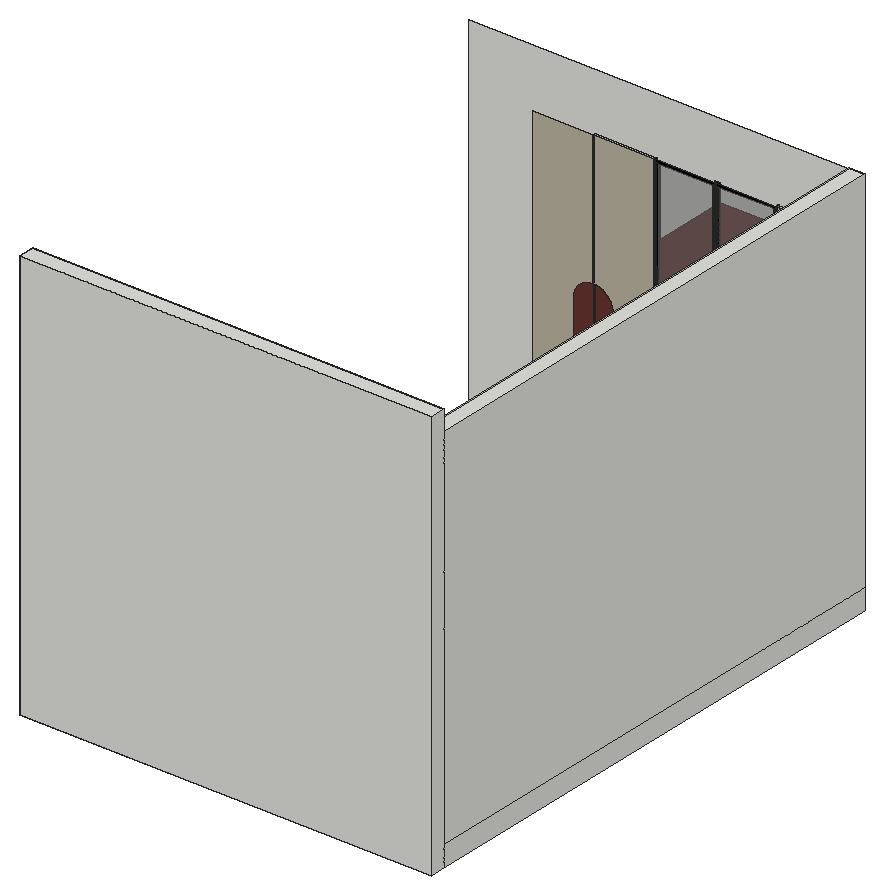
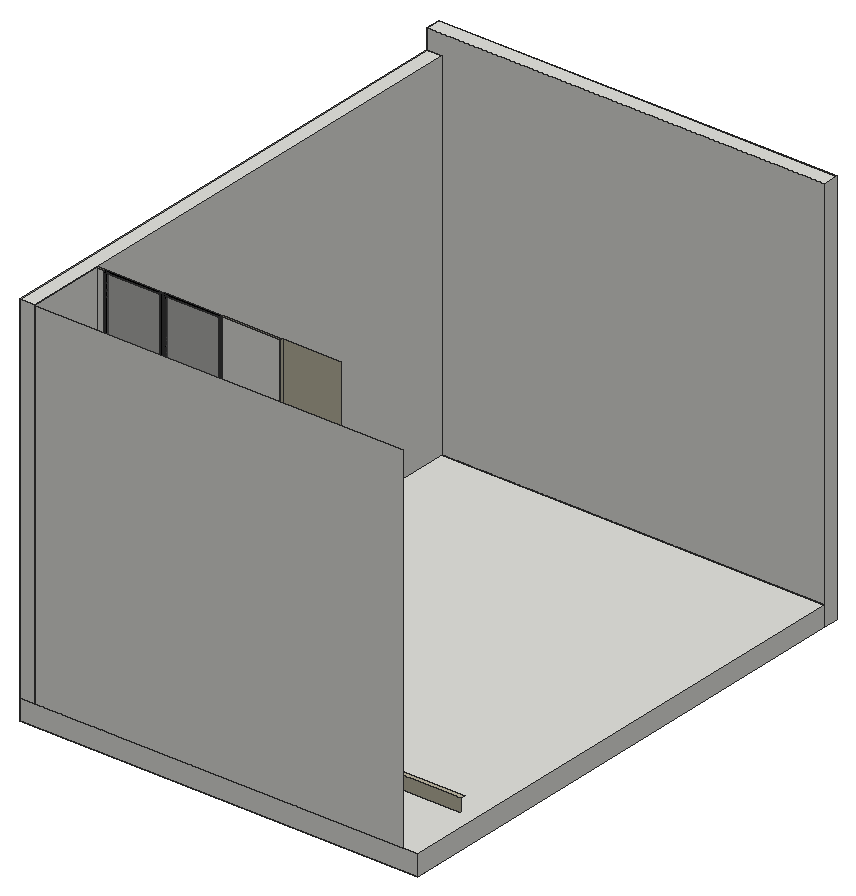
# SketchUp Ruby script. Lengths in millimetres.
U = 1.mm
M = Sketchup.active_model
def pt(a) = Geom::Point3d.new(a.map { |v| v * U })
def face(e, loops, mat)
  f = e.add_face(loops[0].map { |a| pt(a) })
  loops[1..].each { |l| e.add_face(l.map { |a| pt(a) }).erase! }
  f.material = f.back_material = mat if mat
  f
end
# faces: each face lists its corners as indices into pts; further lists are holes
def faces(e, pts, list, mat = nil) = list.each { |f| face(e, (f[0].is_a?(Array) ? f : [f]).map { |l| l.map { |i| pts[i] } }, mat) }
# xy, xz, yz: faces in a plane at the given z, y or x. An outline is a flat list of corners, or four numbers for a rectangle; further outlines are holes
def ring(l) = l.size == 4 ? [[l[0], l[1]], [l[2], l[1]], [l[2], l[3]], [l[0], l[3]]] : l.each_slice(2).to_a
def flat(e, list, mat, &to3) = list.each { |f| face(e, (f[0].is_a?(Array) ? f : [f]).map { |l| ring(l).map { |u, v| to3.(u, v) } }, mat) }
def xy(e, z, list, mat = nil) = flat(e, list, mat) { |x, y| [x, y, z] }
def xz(e, y, list, mat = nil) = flat(e, list, mat) { |x, z| [x, y, z] }
def yz(e, x, list, mat = nil) = flat(e, list, mat) { |y, z| [x, y, z] }
def lines(e, pts, list) = list.each { |a, b| e.add_line(pt(pts[a]), pt(pts[b])) }
# prism: a flat outline (further loops are holes) pulled along v
def prism(e, loops, v, mat = nil)
  f = face(e, loops, mat); d = Geom::Vector3d.new(v.map { |x| x * U })
  f.pushpull(f.normal.samedirection?(d) ? d.length : -d.length)
end
def box(e, o, s, mat = nil) = prism(e, [[o, [o[0] + s[0], o[1], o[2]], [o[0] + s[0], o[1] + s[1], o[2]], [o[0], o[1] + s[1], o[2]]]], [0, 0, s[2]], mat)
def at(x, y, z, deg = 0) = Geom::Transformation.translation(pt([x, y, z])) * Geom::Transformation.rotation(ORIGIN, Z_AXIS, deg.degrees)
def axes(o, x, y, z) = Geom::Transformation.new([*x, 0, *y, 0, *z, 0, *pt(o).to_a, 1])
def part(name) = M.definitions.add(name)
# library, detail: a bought-in or finely detailed component or shape, given as its bounding box
def library(name, o, s) = part(name).tap { |d| box(d.entities, o, s) }
def detail(e, o, s) = box(e.add_group.entities, o, s)
def put(e, d, t, mat = nil) = e.add_instance(d, t).tap { |i| i.material = mat if mat }
def group(e, t, mat = nil) = e.add_group.tap { |g| g.transformation = t; g.material = mat if mat }.entities
root = M.entities
M.materials.add("Uniboard-L17-Ambrette-4K").color = [104, 52, 49]
M.materials.add("Uniboard-L19-Putty-4K").color = [187, 181, 160]
M.materials.add("[Color A07]").color = [153, 0, 0]
M.materials.add("[Color M09]").color = [0, 0, 0]
M.materials.add("[Translucent Glass Gray]").color = [128, 128, 128]
M.materials["[Translucent Glass Gray]"].alpha = 0.5
c1 = part("Group\#4")
box(c1.entities,[0,0,-18],[863.9,559,18])
xy(root,152.4,[[114.3,3454.4,2933.7,4013.2]])
xy(root,254,[[1980,3403.6,2428.4,3421.6],[2431.4,3403.6,2879.9,3421.6],[2882.9,3403.6,2933.7,3421.6]])
xy(root,254,[[1527,3403.6,1977,3421.6],[114.3,3421.6,2933.7,3454.4]],"Uniboard-L19-Putty-4K")
xy(root,268.3,[[1980,3421.6,2879.9,3423.2]])
xy(root,272,[[1980,3423.2,2879.9,3423.2,2879.9,3424.6,2861.9,3424.6,2861.9,3983.6,1998,3983.6,1998,3424.6,1980,3424.6]],"Uniboard-L17-Ambrette-4K")
xy(root,272,[[1998,3403.6,2410.4,3412.6],[2449.4,3403.6,2861.9,3412.6],[1998,3412.6,2410.4,3421.6],[2449.4,3412.6,2861.9,3421.6]],"[Color M09]")
xz(root,3403.6,[[1074,254,1524,254,1524,685.8,1519.2,685.9,1514.4,686.1,1509.7,686.5,1504.9,687,1500.2,687.7,1495.4,688.5,1490.8,689.5,1486.1,690.6,1481.5,691.9,1476.9,693.3,1472.4,694.8,1467.9,696.5,1463.5,698.3,1459.1,700.3,1454.8,702.4,1446.4,707,1442.3,709.5,1438.3,712.2,1434.4,714.9,1430.6,717.8,1426.9,720.8,1423.2,723.9,1419.7,727.1,1416.2,730.4,1412.9,733.9,1409.7,737.4,1406.6,741.1,1403.6,744.8,1400.7,748.6,1398,752.5,1395.3,756.5,1392.8,760.6,1388.2,769,1386.1,773.3,1384.1,777.7,1382.3,782.1,1380.6,786.6,1379.1,791.1,1377.7,795.7,1376.4,800.3,1375.3,805,1374.3,809.6,1373.5,814.4,1372.8,819.1,1372.3,823.9,1371.9,828.6,1371.7,833.4,1371.6,838.2,1371.6,1752.6,1371.7,1757.4,1371.9,1762.2,1372.3,1766.9,1372.8,1771.7,1373.5,1776.4,1374.3,1781.2,1375.3,1785.8,1376.4,1790.5,1377.7,1795.1,1379.1,1799.7,1380.6,1804.2,1382.3,1808.7,1384.1,1813.1,1386.1,1817.5,1388.2,1821.8,1392.8,1830.2,1395.3,1834.3,1398,1838.3,1400.7,1842.2,1403.6,1846,1406.6,1849.7,1409.7,1853.4,1412.9,1856.9,1416.2,1860.4,1419.7,1863.7,1423.2,1866.9,1426.9,1870,1430.6,1873,1434.4,1875.9,1438.3,1878.6,1442.3,1881.3,1446.4,1883.8,1454.8,1888.4,1459.1,1890.5,1463.5,1892.5,1467.9,1894.3,1472.4,1896,1476.9,1897.5,1481.5,1898.9,1486.1,1900.2,1490.8,1901.3,1495.4,1902.3,1500.2,1903.1,1504.9,1903.8,1509.7,1904.3,1514.4,1904.7,1519.2,1904.9,1524,1905,1524,2889.6,1074,2889.6],[1527,254,1977,254,1977,2889.6,1527,2889.6,1527,1905,1528.8,1904.9,1533.6,1904.7,1538.3,1904.3,1543.1,1903.8,1547.8,1903.1,1552.6,1902.3,1557.2,1901.3,1561.9,1900.2,1566.5,1898.9,1571.1,1897.5,1575.6,1896,1580.1,1894.3,1584.5,1892.5,1588.9,1890.5,1593.2,1888.4,1601.6,1883.8,1605.7,1881.3,1609.7,1878.6,1613.6,1875.9,1617.4,1873,1621.1,1870,1624.8,1866.9,1628.3,1863.7,1631.8,1860.4,1635.1,1856.9,1638.3,1853.4,1641.4,1849.7,1644.4,1846,1647.3,1842.2,1650,1838.3,1652.7,1834.3,1655.2,1830.2,1659.8,1821.8,1661.9,1817.5,1663.9,1813.1,1665.7,1808.7,1667.4,1804.2,1668.9,1799.7,1670.3,1795.1,1671.6,1790.5,1672.7,1785.8,1673.7,1781.2,1674.5,1776.4,1675.2,1771.7,1675.7,1766.9,1676.1,1762.2,1676.3,1757.4,1676.4,1752.6,1676.4,838.2,1676.3,833.4,1676.1,828.6,1675.7,823.9,1675.2,819.1,1674.5,814.4,1673.7,809.6,1672.7,805,1671.6,800.3,1670.3,795.7,1668.9,791.1,1667.4,786.6,1665.7,782.1,1663.9,777.7,1661.9,773.3,1659.8,769,1655.2,760.6,1652.7,756.5,1650,752.5,1647.3,748.6,1644.4,744.8,1641.4,741.1,1638.3,737.4,1635.1,733.9,1631.8,730.4,1628.3,727.1,1624.8,723.9,1621.1,720.8,1617.4,717.8,1613.6,714.9,1609.7,712.2,1605.7,709.5,1601.6,707,1593.2,702.4,1588.9,700.3,1584.5,698.3,1580.1,696.5,1575.6,694.8,1571.1,693.3,1566.5,691.9,1561.9,690.6,1557.2,689.5,1552.6,688.5,1547.8,687.7,1543.1,687,1538.3,686.5,1533.6,686.1,1528.8,685.9,1527,685.8],[2882.9,254,2933.7,2889.6]],"Uniboard-L19-Putty-4K")
xz(root,3403.6,[[[1980,254,2428.4,2889.6],[1998,272,2410.4,2871.6]],[[2431.4,254,2879.9,2889.6],[2449.4,272,2861.9,2871.6]]],"[Color M09]")
xz(root,3412.6,[[1998,272,2410.4,2871.6],[2449.4,272,2861.9,2871.6]],"[Translucent Glass Gray]")
xz(root,3413.6,[[1524,685.8,1524,1217.7,1523.1,1217.7,1520.6,1217.9,1518.2,1218,1515.8,1218.3,1513.3,1218.7,1510.3,1219.2,1508.6,1219.6,1506.2,1220.1,1503.8,1220.8,1501.5,1221.5,1499.2,1222.3,1494.6,1224.1,1492.4,1225.1,1490.2,1226.2,1488.1,1227.3,1485.9,1228.5,1483.9,1229.8,1481.8,1231.1,1479.8,1232.5,1476,1235.5,1474.1,1237.1,1472.3,1238.8,1468.9,1242.2,1467.2,1244,1465.6,1245.9,1462.6,1249.7,1461.2,1251.7,1459.9,1253.8,1458.6,1255.8,1457.4,1258,1456.3,1260.1,1455.2,1262.3,1454.2,1264.5,1452.4,1269.1,1451.6,1271.4,1450.9,1273.7,1450.2,1276.1,1449.7,1278.5,1449.2,1280.8,1448.8,1283.2,1448.4,1285.7,1448.1,1288.1,1448,1290.5,1447.8,1293,1447.8,1297.8,1448,1300.3,1448.1,1302.7,1448.4,1305.1,1448.8,1307.6,1449.2,1310,1449.7,1312.3,1450.2,1314.7,1450.9,1317.1,1451.6,1319.4,1452.4,1321.7,1454.2,1326.3,1455.2,1328.5,1456.3,1330.7,1457.4,1332.8,1458.6,1335,1459.9,1337,1461.2,1339.1,1462.6,1341.1,1465.6,1344.9,1467.2,1346.8,1468.9,1348.6,1472.3,1352,1474.1,1353.7,1476,1355.3,1479.8,1358.3,1481.8,1359.7,1483.9,1361,1485.9,1362.3,1488.1,1363.5,1490.2,1364.6,1492.4,1365.7,1494.6,1366.7,1499.2,1368.5,1501.5,1369.3,1503.8,1370,1506.2,1370.7,1508.6,1371.2,1510.3,1371.6,1513.3,1372.1,1515.8,1372.5,1518.2,1372.8,1520.6,1372.9,1523.1,1373.1,1524,1373.1,1524,1905,1519.2,1904.9,1514.4,1904.7,1509.7,1904.3,1504.9,1903.8,1500.2,1903.1,1495.4,1902.3,1490.8,1901.3,1486.1,1900.2,1481.5,1898.9,1476.9,1897.5,1472.4,1896,1467.9,1894.3,1463.5,1892.5,1459.1,1890.5,1454.8,1888.4,1446.4,1883.8,1442.3,1881.3,1438.3,1878.6,1434.4,1875.9,1430.6,1873,1426.9,1870,1423.2,1866.9,1419.7,1863.7,1416.2,1860.4,1412.9,1856.9,1409.7,1853.4,1406.6,1849.7,1403.6,1846,1400.7,1842.2,1398,1838.3,1395.3,1834.3,1392.8,1830.2,1388.2,1821.8,1386.1,1817.5,1384.1,1813.1,1382.3,1808.7,1380.6,1804.2,1379.1,1799.7,1377.7,1795.1,1376.4,1790.5,1375.3,1785.8,1374.3,1781.2,1373.5,1776.4,1372.8,1771.7,1372.3,1766.9,1371.9,1762.2,1371.7,1757.4,1371.6,1752.6,1371.6,838.2,1371.7,833.4,1371.9,828.6,1372.3,823.9,1372.8,819.1,1373.5,814.4,1374.3,809.6,1375.3,805,1376.4,800.3,1377.7,795.7,1379.1,791.1,1380.6,786.6,1382.3,782.1,1384.1,777.7,1386.1,773.3,1388.2,769,1392.8,760.6,1395.3,756.5,1398,752.5,1400.7,748.6,1403.6,744.8,1406.6,741.1,1409.7,737.4,1412.9,733.9,1416.2,730.4,1419.7,727.1,1423.2,723.9,1426.9,720.8,1430.6,717.8,1434.4,714.9,1438.3,712.2,1442.3,709.5,1446.4,707,1454.8,702.4,1459.1,700.3,1463.5,698.3,1467.9,696.5,1472.4,694.8,1476.9,693.3,1481.5,691.9,1486.1,690.6,1490.8,689.5,1495.4,688.5,1500.2,687.7,1504.9,687,1509.7,686.5,1514.4,686.1,1519.2,685.9],[1527,685.8,1528.8,685.9,1533.6,686.1,1538.3,686.5,1543.1,687,1547.8,687.7,1552.6,688.5,1557.2,689.5,1561.9,690.6,1566.5,691.9,1571.1,693.3,1575.6,694.8,1580.1,696.5,1584.5,698.3,1588.9,700.3,1593.2,702.4,1601.6,707,1605.7,709.5,1609.7,712.2,1613.6,714.9,1617.4,717.8,1621.1,720.8,1624.8,723.9,1628.3,727.1,1631.8,730.4,1635.1,733.9,1638.3,737.4,1641.4,741.1,1644.4,744.8,1647.3,748.6,1650,752.5,1652.7,756.5,1655.2,760.6,1659.8,769,1661.9,773.3,1663.9,777.7,1665.7,782.1,1667.4,786.6,1668.9,791.1,1670.3,795.7,1671.6,800.3,1672.7,805,1673.7,809.6,1674.5,814.4,1675.2,819.1,1675.7,823.9,1676.1,828.6,1676.3,833.4,1676.4,838.2,1676.4,1752.6,1676.3,1757.4,1676.1,1762.2,1675.7,1766.9,1675.2,1771.7,1674.5,1776.4,1673.7,1781.2,1672.7,1785.8,1671.6,1790.5,1670.3,1795.1,1668.9,1799.7,1667.4,1804.2,1665.7,1808.7,1663.9,1813.1,1661.9,1817.5,1659.8,1821.8,1655.2,1830.2,1652.7,1834.3,1650,1838.3,1647.3,1842.2,1644.4,1846,1641.4,1849.7,1638.3,1853.4,1635.1,1856.9,1631.8,1860.4,1628.3,1863.7,1624.8,1866.9,1621.1,1870,1617.4,1873,1613.6,1875.9,1609.7,1878.6,1605.7,1881.3,1601.6,1883.8,1593.2,1888.4,1588.9,1890.5,1584.5,1892.5,1580.1,1894.3,1575.6,1896,1571.1,1897.5,1566.5,1898.9,1561.9,1900.2,1557.2,1901.3,1552.6,1902.3,1547.8,1903.1,1543.1,1903.8,1538.3,1904.3,1533.6,1904.7,1528.8,1904.9,1527,1905,1527,1373.1,1527.9,1373.1,1530.4,1372.9,1532.8,1372.8,1535.2,1372.5,1537.7,1372.1,1540.7,1371.6,1542.4,1371.2,1544.8,1370.7,1547.2,1370,1549.5,1369.3,1551.8,1368.5,1556.4,1366.7,1558.6,1365.7,1560.8,1364.6,1562.9,1363.5,1565.1,1362.3,1567.1,1361,1569.2,1359.7,1571.2,1358.3,1575,1355.3,1576.9,1353.7,1578.7,1352,1582.1,1348.6,1583.8,1346.8,1585.4,1344.9,1588.4,1341.1,1589.8,1339.1,1591.1,1337,1592.4,1335,1593.6,1332.8,1594.7,1330.7,1595.8,1328.5,1596.8,1326.3,1598.6,1321.7,1599.4,1319.4,1600.1,1317.1,1600.8,1314.7,1601.3,1312.3,1601.8,1310,1602.2,1307.6,1602.6,1305.1,1602.9,1302.7,1603,1300.3,1603.2,1297.8,1603.2,1293,1603,1290.5,1602.9,1288.1,1602.6,1285.7,1602.2,1283.2,1601.8,1280.8,1601.3,1278.5,1600.8,1276.1,1600.1,1273.7,1599.4,1271.4,1598.6,1269.1,1596.8,1264.5,1595.8,1262.3,1594.7,1260.1,1593.6,1258,1592.4,1255.8,1591.1,1253.8,1589.8,1251.7,1588.4,1249.7,1585.4,1245.9,1583.8,1244,1582.1,1242.2,1578.7,1238.8,1576.9,1237.1,1575,1235.5,1571.2,1232.5,1569.2,1231.1,1567.1,1229.8,1565.1,1228.5,1562.9,1227.3,1560.8,1226.2,1558.6,1225.1,1556.4,1224.1,1551.8,1222.3,1549.5,1221.5,1547.2,1220.8,1544.8,1220.1,1542.4,1219.6,1540.7,1219.2,1537.7,1218.7,1535.2,1218.3,1532.8,1218,1530.4,1217.9,1527.9,1217.7,1527,1217.7]],"Uniboard-L17-Ambrette-4K")
xz(root,3421.6,[[1527,254,1977,2889.6],[1980,254,2428.4,268.3],[2428.4,254,2431.4,268.3],[2431.4,254,2879.9,268.3],[2882.9,254,2933.7,2889.6],
  [1980,268.3,2410.4,272],[1980,272,1998,2871.6]])
xz(root,3421.6,[[1524,254,1527,2889.6],[1977,254,1980,2889.6],[2879.9,254,2882.9,2889.6]],"Uniboard-L19-Putty-4K")
xz(root,3421.6,[[2410.4,268.3,2428.4,2889.6],[2431.4,268.3,2449.4,2889.6],[2449.4,268.3,2879.9,272],[2861.9,272,2879.9,2871.6]],"[Color M09]")
xz(root,3423.2,[[1980,268.3,2410.4,272],[2410.4,268.3,2428.4,272],[2428.4,268.3,2431.4,272],[2431.4,268.3,2449.4,272]])
xz(root,3423.2,[[2449.4,268.3,2879.9,272]],"[Color A07]")
xz(root,3424.6,[[1980,272,1998,2871.6],[2861.9,272,2879.9,2871.6]],"[Color A07]")
xz(root,3454.4,[[114.3,152.4,2933.7,254]],"Uniboard-L19-Putty-4K")
xz(root,3983.6,[[1998,272,2861.9,2351.7]],"Uniboard-L17-Ambrette-4K")
xz(root,4013.2,[[114.3,152.4,2933.7,2889.6]])
yz(root,1524,[[3403.6,254,3421.6,254,3421.6,2889.6,3403.6,2889.6,3403.6,1905,3413.6,1905,3413.6,685.8,3403.6,685.8]],"Uniboard-L19-Putty-4K")
yz(root,1527,[[3403.6,254,3403.6,685.8,3413.6,685.8,3413.6,1905,3403.6,1905,3403.6,2889.6,3421.6,2889.6,3421.6,254]],"Uniboard-L19-Putty-4K")
yz(root,1676.4,[[3403.6,838.2,3413.6,1752.6]],"Uniboard-L17-Ambrette-4K")
yz(root,1977,[[3403.6,254,3421.6,2889.6]],"Uniboard-L19-Putty-4K")
yz(root,1980,[[3421.6,268.3,3423.2,268.3,3423.2,272,3424.6,272,3424.6,2889.6,3421.6,2889.6]])
yz(root,1980,[[3403.6,254,3421.6,2889.6]],"[Color M09]")
yz(root,1998,[[3424.6,272,3983.6,2351.7]],"Uniboard-L17-Ambrette-4K")
yz(root,1998,[[3403.6,272,3412.6,2871.6],[3412.6,272,3421.6,2871.6]],"[Color M09]")
yz(root,2410.4,[[3403.6,272,3412.6,2871.6],[3412.6,272,3421.6,2871.6]],"[Color M09]")
yz(root,2428.4,[[3403.6,254,3421.6,2889.6]],"[Color M09]")
yz(root,2431.4,[[3403.6,254,3421.6,2889.6]],"[Color M09]")
yz(root,2449.4,[[3403.6,272,3412.6,2871.6],[3412.6,272,3421.6,2871.6]],"[Color M09]")
yz(root,2861.9,[[3424.6,272,3983.6,2351.7]],"Uniboard-L17-Ambrette-4K")
yz(root,2861.9,[[3403.6,272,3412.6,2871.6],[3412.6,272,3421.6,2871.6]],"[Color M09]")
yz(root,2879.9,[[3421.6,268.3,3421.6,2889.6,3424.6,2889.6,3424.6,272,3423.2,272,3423.2,268.3]])
yz(root,2879.9,[[3403.6,254,3421.6,2889.6]],"[Color M09]")
yz(root,2882.9,[[3403.6,254,3421.6,2889.6]],"Uniboard-L19-Putty-4K")
yz(root,2933.7,[[3454.4,152.4,4013.2,152.4,4013.2,2889.6,3421.6,2889.6,3421.6,254,3454.4,254],[3403.6,254,3421.6,2889.6]])
p = [[1519.2,3403.6,685.9],[1524,3403.6,685.8],[1524,3413.6,685.8],[1519.2,3413.6,685.9],[1527,3403.6,685.8],[1528.8,3403.6,685.9],
  [1528.8,3413.6,685.9],[1527,3413.6,685.8],[1514.4,3403.6,686.1],[1514.4,3413.6,686.1],[1533.6,3403.6,686.1],[1533.6,3413.6,686.1],
  [1509.7,3403.6,686.5],[1509.7,3413.6,686.5],[1538.3,3403.6,686.5],[1538.3,3413.6,686.5],[1504.9,3403.6,687],[1504.9,3413.6,687],
  [1543.1,3403.6,687],[1543.1,3413.6,687],[1500.2,3403.6,687.7],[1500.2,3413.6,687.7],[1547.8,3403.6,687.7],[1547.8,3413.6,687.7],
  [1495.4,3403.6,688.5],[1495.4,3413.6,688.5],[1552.6,3403.6,688.5],[1552.6,3413.6,688.5],[1490.8,3403.6,689.5],[1490.8,3413.6,689.5],
  [1557.2,3403.6,689.5],[1557.2,3413.6,689.5],[1486.1,3403.6,690.6],[1486.1,3413.6,690.6],[1561.9,3403.6,690.6],[1561.9,3413.6,690.6],
  [1481.5,3403.6,691.9],[1481.5,3413.6,691.9],[1566.5,3403.6,691.9],[1566.5,3413.6,691.9],[1476.9,3403.6,693.3],[1476.9,3413.6,693.3],
  [1571.1,3403.6,693.3],[1571.1,3413.6,693.3],[1472.4,3403.6,694.8],[1472.4,3413.6,694.8],[1575.6,3403.6,694.8],[1575.6,3413.6,694.8],
  [1467.9,3403.6,696.5],[1467.9,3413.6,696.5],[1580.1,3403.6,696.5],[1580.1,3413.6,696.5],[1463.5,3403.6,698.3],[1463.5,3413.6,698.3],
  [1584.5,3403.6,698.3],[1584.5,3413.6,698.3],[1459.1,3403.6,700.3],[1459.1,3413.6,700.3],[1588.9,3403.6,700.3],[1588.9,3413.6,700.3],
  [1454.8,3403.6,702.4],[1454.8,3413.6,702.4],[1593.2,3403.6,702.4],[1593.2,3413.6,702.4],[1450.6,3403.6,704.7],[1450.6,3413.6,704.7],
  [1597.4,3403.6,704.7],[1597.4,3413.6,704.7],[1446.4,3403.6,707],[1446.4,3413.6,707],[1601.6,3403.6,707],[1601.6,3413.6,707],
  [1442.3,3403.6,709.5],[1442.3,3413.6,709.5],[1605.7,3403.6,709.5],[1605.7,3413.6,709.5],[1438.3,3403.6,712.2],[1438.3,3413.6,712.2],
  [1609.7,3403.6,712.2],[1609.7,3413.6,712.2],[1434.4,3403.6,714.9],[1434.4,3413.6,714.9],[1613.6,3403.6,714.9],[1613.6,3413.6,714.9],
  [1430.6,3403.6,717.8],[1430.6,3413.6,717.8],[1617.4,3403.6,717.8],[1617.4,3413.6,717.8],[1426.9,3403.6,720.8],[1426.9,3413.6,720.8],
  [1621.1,3403.6,720.8],[1621.1,3413.6,720.8],[1423.2,3403.6,723.9],[1423.2,3413.6,723.9],[1624.8,3403.6,723.9],[1624.8,3413.6,723.9],
  [1419.7,3403.6,727.1],[1419.7,3413.6,727.1],[1628.3,3403.6,727.1],[1628.3,3413.6,727.1],[1416.2,3403.6,730.4],[1416.2,3413.6,730.4],
  [1631.8,3403.6,730.4],[1631.8,3413.6,730.4],[1412.9,3403.6,733.9],[1412.9,3413.6,733.9],[1635.1,3403.6,733.9],[1635.1,3413.6,733.9],
  [1409.7,3403.6,737.4],[1409.7,3413.6,737.4],[1638.3,3403.6,737.4],[1638.3,3413.6,737.4],[1406.6,3403.6,741.1],[1406.6,3413.6,741.1],
  [1641.4,3403.6,741.1],[1641.4,3413.6,741.1],[1403.6,3403.6,744.8],[1403.6,3413.6,744.8],[1644.4,3403.6,744.8],[1644.4,3413.6,744.8],
  [1647.3,3403.6,748.6],[1647.3,3413.6,748.6],[1650,3403.6,752.5],[1650,3413.6,752.5],[1652.7,3403.6,756.5],[1652.7,3413.6,756.5],
  [1655.2,3403.6,760.6],[1655.2,3413.6,760.6],[1657.5,3403.6,764.8],[1657.5,3413.6,764.8],[1659.8,3403.6,769],[1659.8,3413.6,769],
  [1661.9,3403.6,773.3],[1661.9,3413.6,773.3],[1663.9,3403.6,777.7],[1663.9,3413.6,777.7],[1665.7,3403.6,782.1],[1665.7,3413.6,782.1],
  [1667.4,3403.6,786.6],[1667.4,3413.6,786.6],[1668.9,3403.6,791.1],[1668.9,3413.6,791.1],[1670.3,3403.6,795.7],[1670.3,3413.6,795.7],
  [1671.6,3403.6,800.3],[1671.6,3413.6,800.3],[1672.7,3403.6,805],[1672.7,3413.6,805],[1673.7,3403.6,809.6],[1673.7,3413.6,809.6],
  [1674.5,3403.6,814.4],[1674.5,3413.6,814.4],[1675.2,3403.6,819.1],[1675.2,3413.6,819.1],[1675.7,3403.6,823.9],[1675.7,3413.6,823.9],
  [1676.1,3403.6,828.6],[1676.1,3413.6,828.6],[1676.3,3403.6,833.4],[1676.3,3413.6,833.4],[1676.4,3403.6,838.2],[1676.4,3413.6,838.2]]
faces(root,p,[[0,1,2,3],[4,5,6,7],[8,0,3,9],[5,10,11,6],[12,8,9,13],[10,14,15,11],[16,12,13,17],[14,18,19,15],
  [20,16,17,21],[18,22,23,19],[24,20,21,25],[22,26,27,23],[28,24,25,29],[26,30,31,27],[32,28,29,33],[30,34,35,31],
  [36,32,33,37],[34,38,39,35],[40,36,37,41],[38,42,43,39],[44,40,41,45],[42,46,47,43],[48,44,45,49],[46,50,51,47],
  [52,48,49,53],[50,54,55,51],[56,52,53,57],[54,58,59,55],[60,56,57,61],[58,62,63,59],[64,60,61,65],[62,66,67,63],
  [68,64,65,69],[66,70,71,67],[72,68,69,73],[70,74,75,71],[76,72,73,77],[74,78,79,75],[80,76,77,81],[78,82,83,79],
  [84,80,81,85],[82,86,87,83],[88,84,85,89],[86,90,91,87],[92,88,89,93],[90,94,95,91],[96,92,93,97],[94,98,99,95],
  [100,96,97,101],[98,102,103,99],[104,100,101,105],[102,106,107,103],[108,104,105,109],[106,110,111,107],[112,108,109,113],[110,114,115,111],
  [116,112,113,117],[114,118,119,115],[118,120,121,119],[120,122,123,121],[122,124,125,123],[124,126,127,125],[126,128,129,127],[128,130,131,129],
  [130,132,133,131],[132,134,135,133],[134,136,137,135],[136,138,139,137],[138,140,141,139],[140,142,143,141],[142,144,145,143],[144,146,147,145],
  [146,148,149,147],[148,150,151,149],[150,152,153,151],[152,154,155,153],[154,156,157,155],[156,158,159,157],[158,160,161,159]],"Uniboard-L17-Ambrette-4K")
g1 = group(root,at(0,965.2,0))
xy(g1,0,[[0,-965.2,3048,-850.9],[0,-850.9,3048,3048]])
xy(g1,152.4,[[0,-850.9,3048,3048]])
xy(g1,3048,[[0,-965.2,3048,-850.9]])
xz(g1,-965.2,[[0,0,3048,3048]])
xz(g1,-850.9,[[0,0,3048,152.4],[0,152.4,3048,3048]])
xz(g1,3048,[[0,0,3048,152.4]])
yz(g1,0,[[-965.2,0,-850.9,3048],[-850.9,0,3048,152.4]])
yz(g1,3048,[[-965.2,0,-850.9,3048],[-850.9,0,3048,152.4]])
put(root,c1,at(1998,3424.6,845.9),"Uniboard-L17-Ambrette-4K")
g2 = group(root,at(2933.7,965.2,152.4))
box(g2,[0,-850.9,0],[114.3,3898.9,2743.2])
